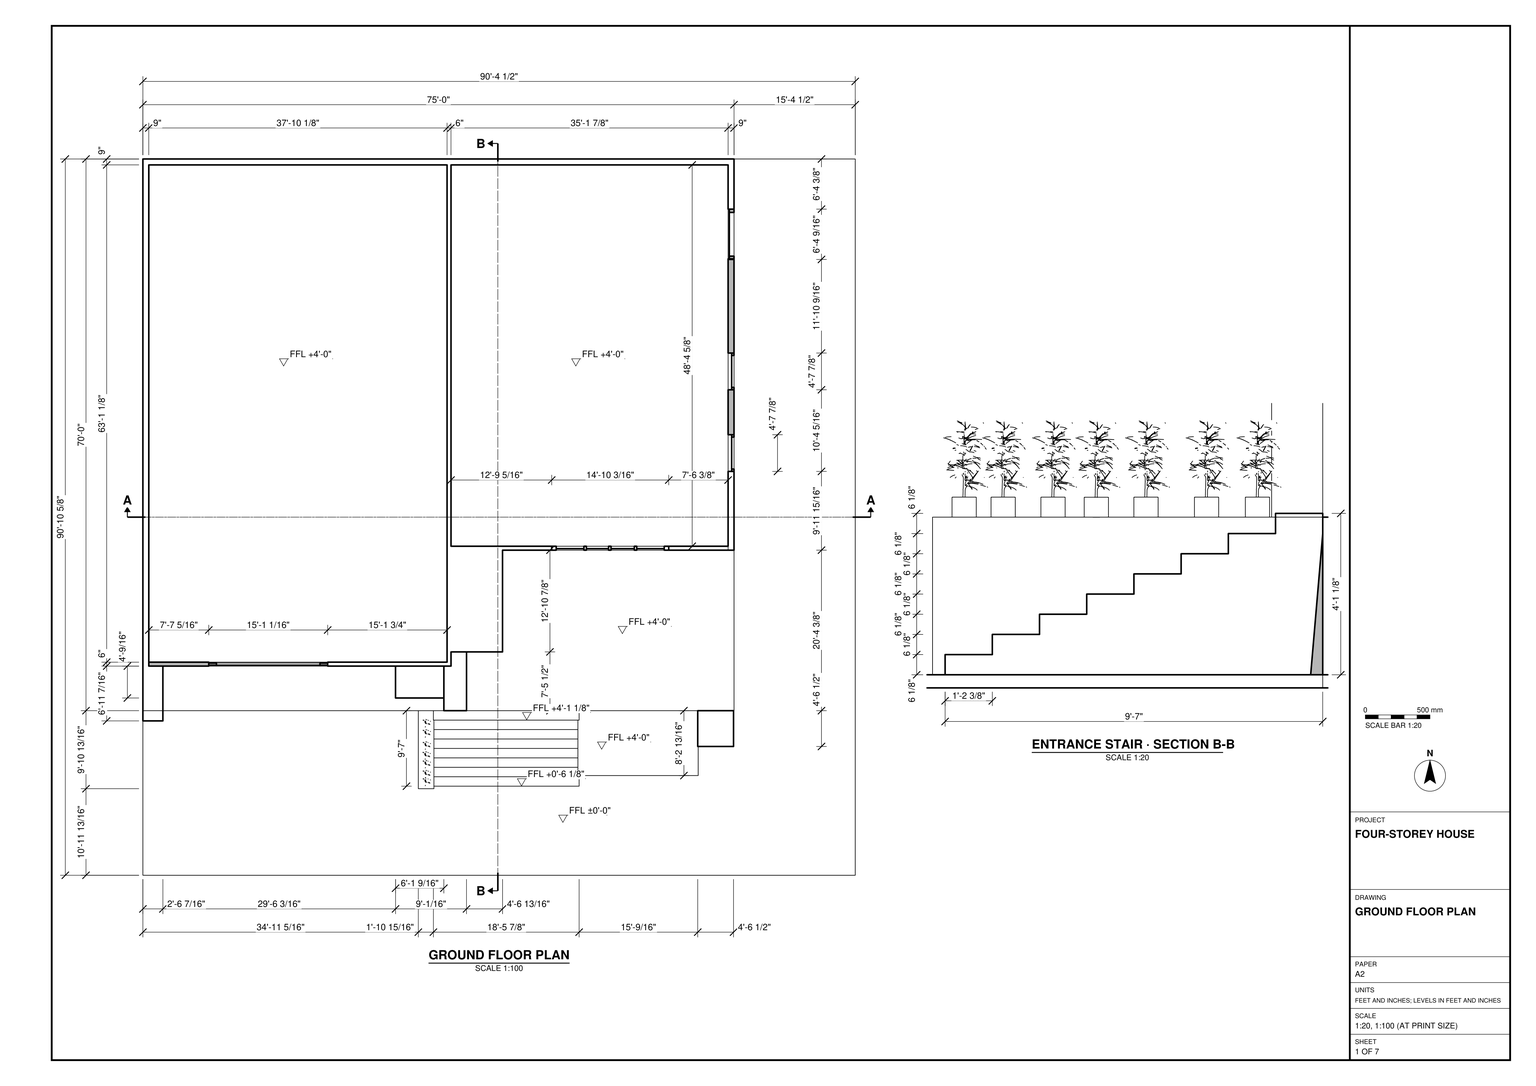
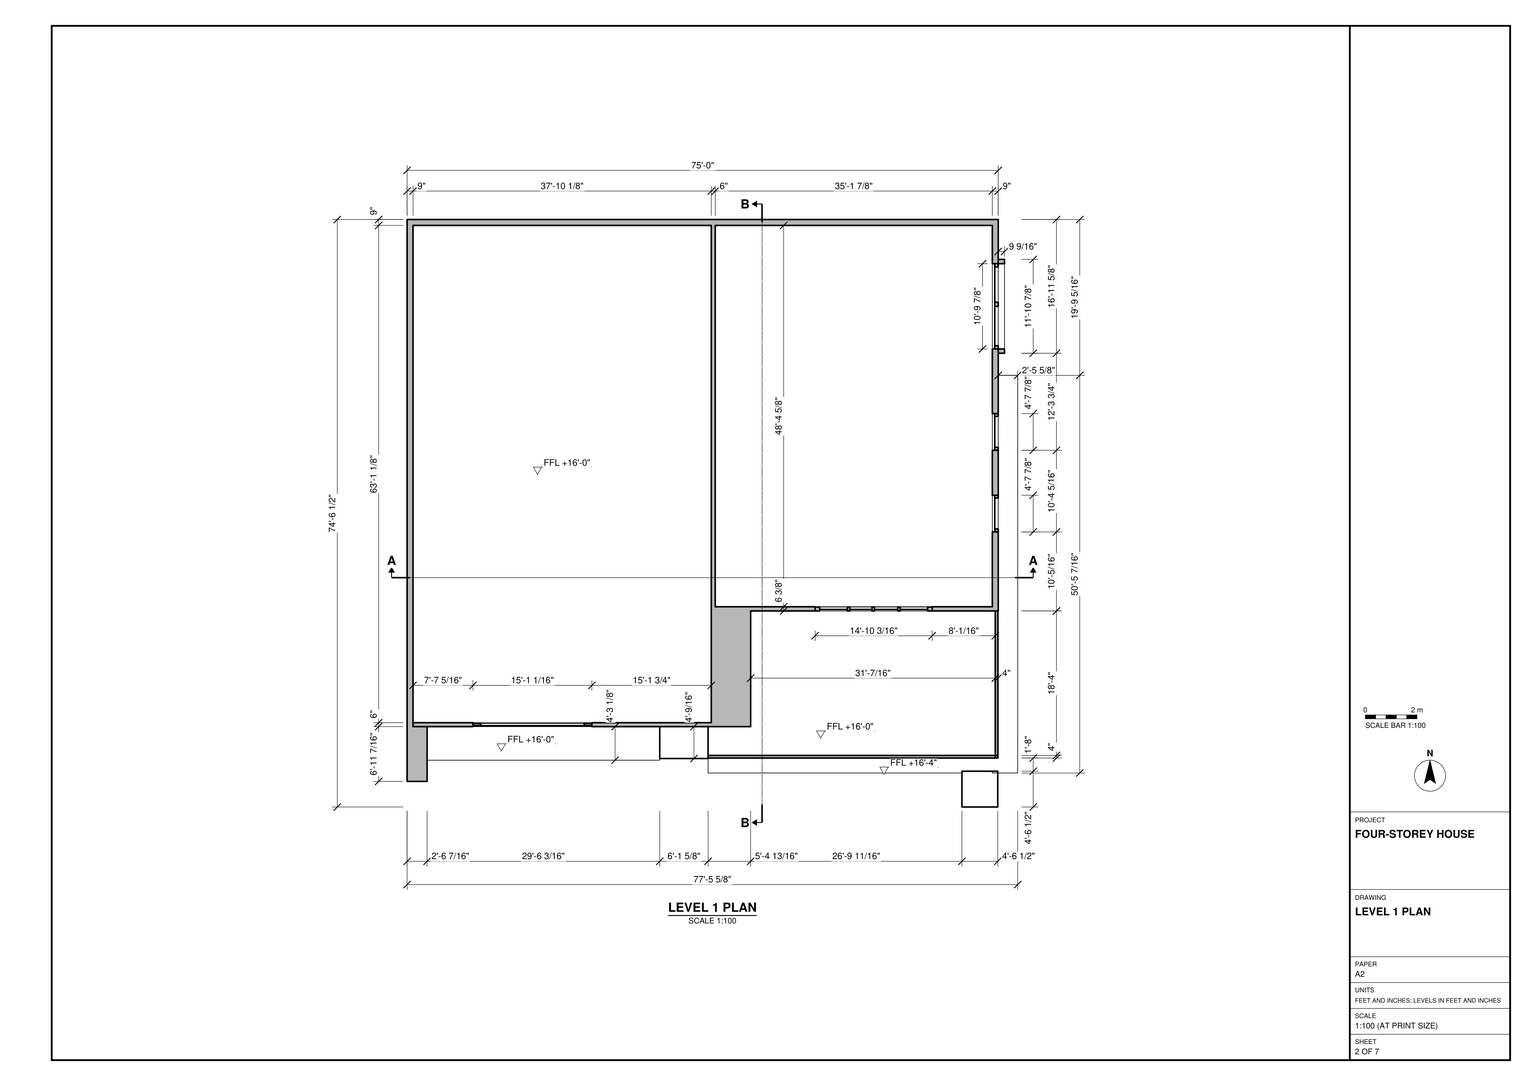
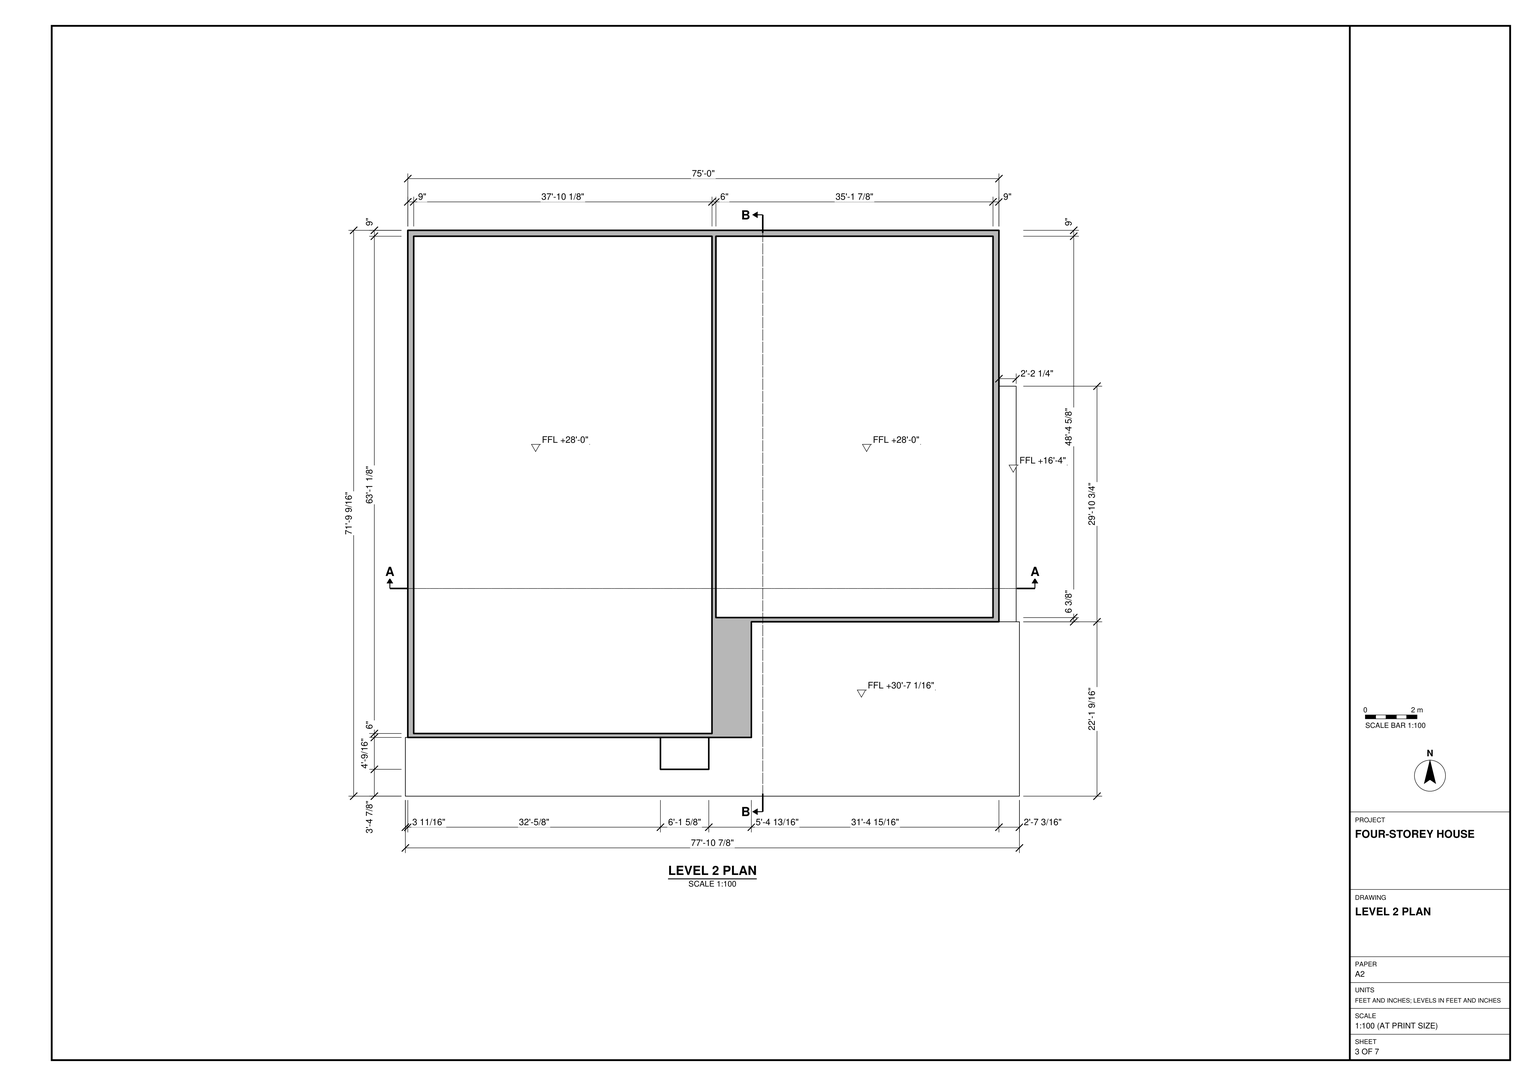
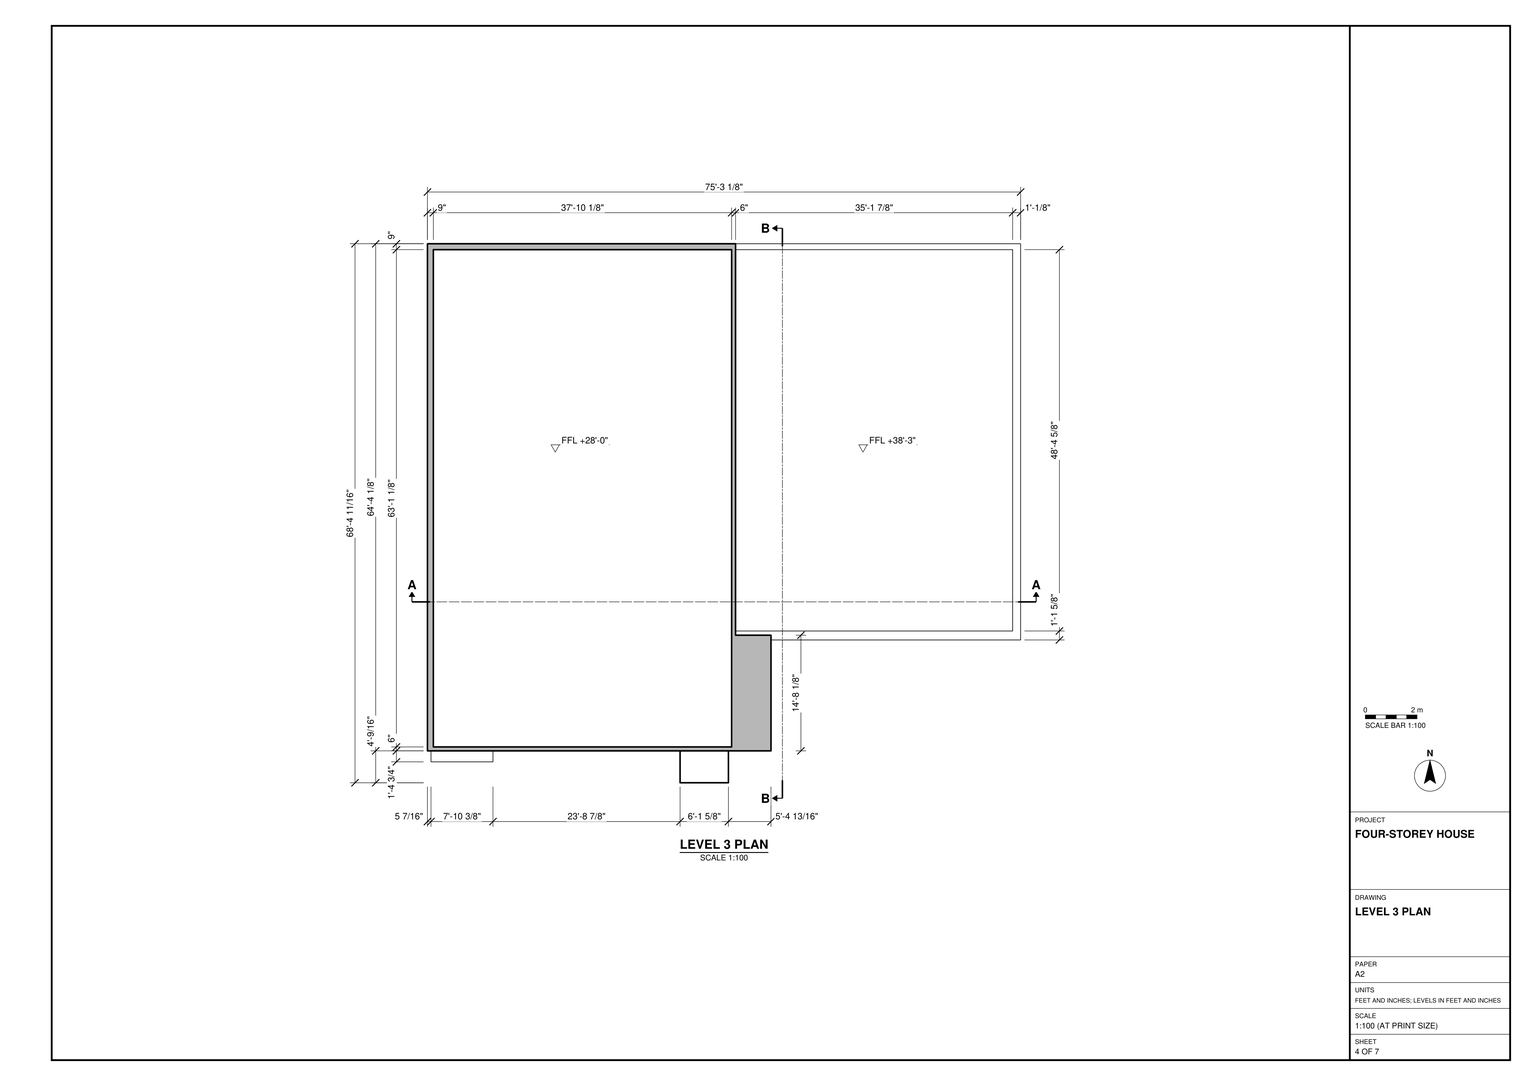
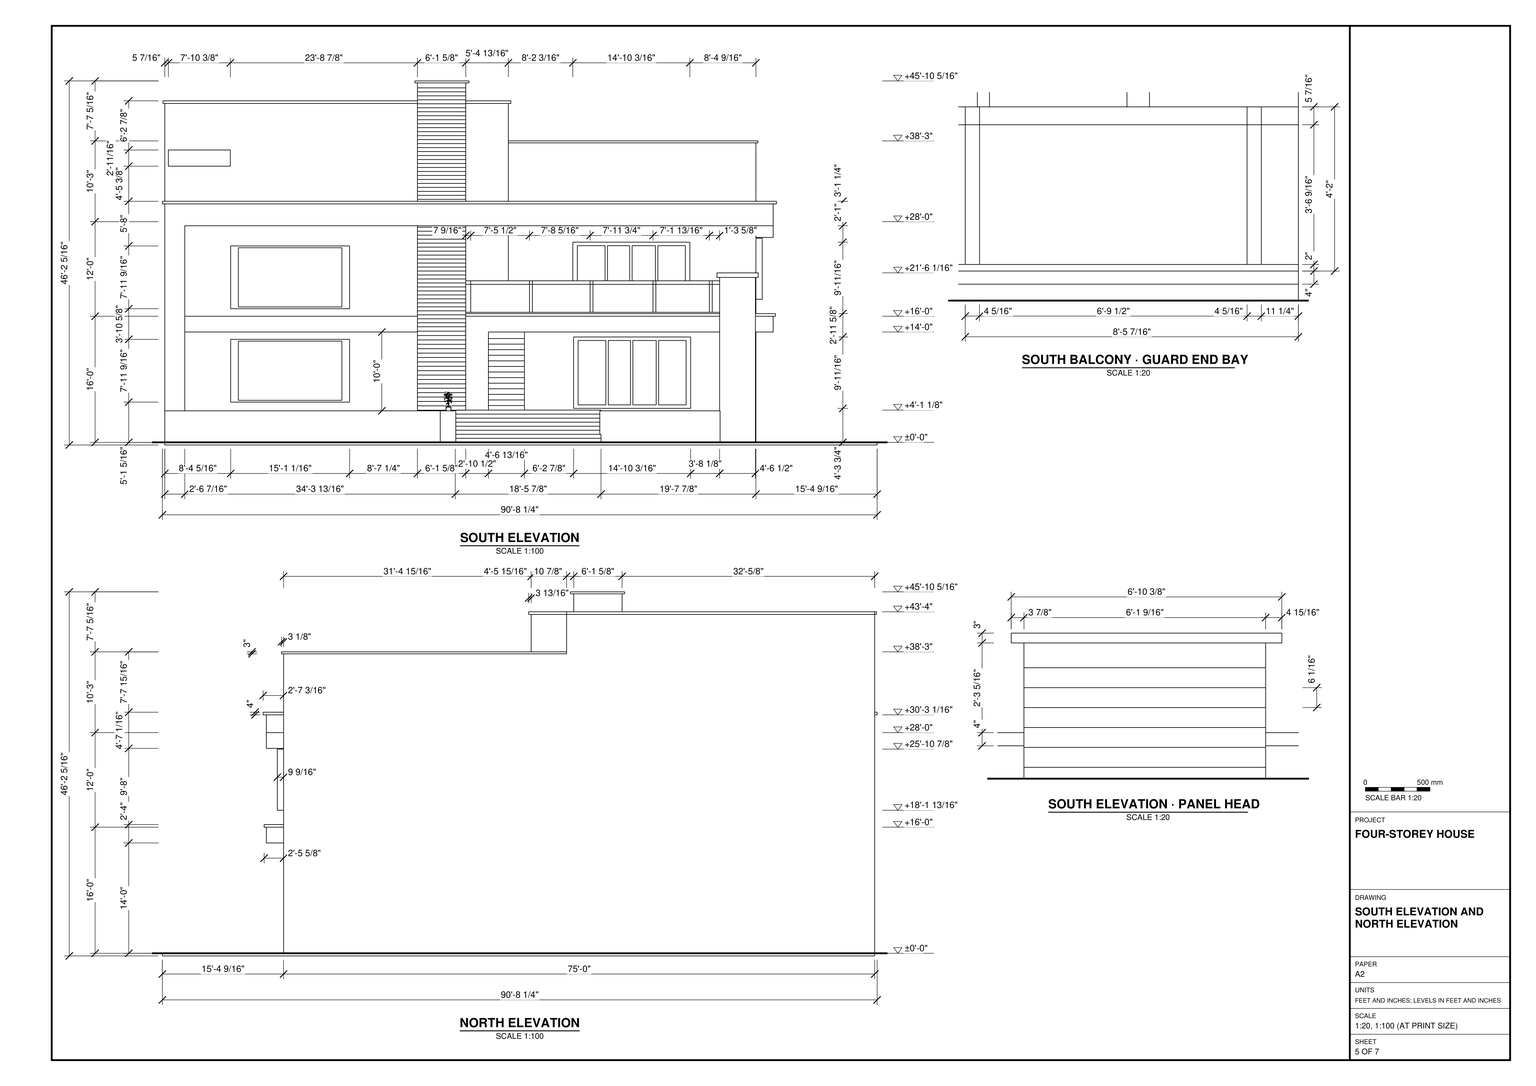
Build the four-storey house and its site in SketchUp from task_files/diagram_01.pdf. Work in feet and inches. Including the site, the model must measure 90'-8 1/4" along X, 90'-10 5/8" along Y and 46'-2 5/16" along Z. Use the level references ±0'-0", +16'-0", +28'-0" and +38'-3". Distinguish the ±0'-0" site datum from the raised ground-floor surface at +4'-0".

Align the two main bays along their rear wall, with the left bay extending farther toward the entrance than the right bay. Use the wall thicknesses shown, including the 9" rear wall and 6" dividing wall. Place the front and side openings in their dimensioned positions. Follow each floor plan for the slab edges, including the terrace in front of the recessed right bay at Level 1. Model the supports and roof to the profiles shown. Use section B-B to form the entrance stair and landing, and place the potted plants along the indicated edge of the stair.

Keep shell elements such as walls, slabs and roof, and each furniture or joinery piece shown, in separate groups or components. Use components for repeated parts. Decor and loose items, including the plants, may be any suitable library components. Save one SketchUp model as output_files/four_storey_house_with_a_raised_entrance.skp.

# SketchUp Ruby script. Lengths in inches.
U = 1.inch
M = Sketchup.active_model
def pt(a) = Geom::Point3d.new(a.map { |v| v * U })
def face(e, loops, mat)
  f = e.add_face(loops[0].map { |a| pt(a) })
  loops[1..].each { |l| e.add_face(l.map { |a| pt(a) }).erase! }
  f.material = f.back_material = mat if mat
  f
end
# faces: each face lists its corners as indices into pts; further lists are holes
def faces(e, pts, list, mat = nil) = list.each { |f| face(e, (f[0].is_a?(Array) ? f : [f]).map { |l| l.map { |i| pts[i] } }, mat) }
# xy, xz, yz: faces in a plane at the given z, y or x. An outline is a flat list of corners, or four numbers for a rectangle; further outlines are holes
def ring(l) = l.size == 4 ? [[l[0], l[1]], [l[2], l[1]], [l[2], l[3]], [l[0], l[3]]] : l.each_slice(2).to_a
def flat(e, list, mat, &to3) = list.each { |f| face(e, (f[0].is_a?(Array) ? f : [f]).map { |l| ring(l).map { |u, v| to3.(u, v) } }, mat) }
def xy(e, z, list, mat = nil) = flat(e, list, mat) { |x, y| [x, y, z] }
def xz(e, y, list, mat = nil) = flat(e, list, mat) { |x, z| [x, y, z] }
def yz(e, x, list, mat = nil) = flat(e, list, mat) { |y, z| [x, y, z] }
def lines(e, pts, list) = list.each { |a, b| e.add_line(pt(pts[a]), pt(pts[b])) }
# prism: a flat outline (further loops are holes) pulled along v
def prism(e, loops, v, mat = nil)
  f = face(e, loops, mat); d = Geom::Vector3d.new(v.map { |x| x * U })
  f.pushpull(f.normal.samedirection?(d) ? d.length : -d.length)
end
def box(e, o, s, mat = nil) = prism(e, [[o, [o[0] + s[0], o[1], o[2]], [o[0] + s[0], o[1] + s[1], o[2]], [o[0], o[1] + s[1], o[2]]]], [0, 0, s[2]], mat)
def at(x, y, z, deg = 0) = Geom::Transformation.translation(pt([x, y, z])) * Geom::Transformation.rotation(ORIGIN, Z_AXIS, deg.degrees)
def axes(o, x, y, z) = Geom::Transformation.new([*x, 0, *y, 0, *z, 0, *pt(o).to_a, 1])
def part(name) = M.definitions.add(name)
# library, detail: a bought-in or finely detailed component or shape, given as its bounding box
def library(name, o, s) = part(name).tap { |d| box(d.entities, o, s) }
def detail(e, o, s) = box(e.add_group.entities, o, s)
def put(e, d, t, mat = nil) = e.add_instance(d, t).tap { |i| i.material = mat if mat }
def group(e, t, mat = nil) = e.add_group.tap { |g| g.transformation = t; g.material = mat if mat }.entities
root = M.entities
M.materials.add("[Color B08]1").color = [50, 25, 0]
M.materials.add("[Color C08]").color = [60, 37, 47]
M.materials.add("[Color M04]").color = [142, 142, 142]
M.materials.add("[Color M05]").color = [114, 114, 114]
M.materials.add("[Color M06]").color = [86, 86, 86]
M.materials.add("[Color M07]").color = [58, 58, 58]
M.materials.add("[Concrete Block Retaining Gray]").color = [121, 121, 121]
M.materials.add("[Pavers with Grass Herringbone]").color = [197, 201, 190]
M.materials.add("[Translucent Glass Gray]").color = [128, 128, 128]
M.materials["[Translucent Glass Gray]"].alpha = 0.5
M.materials.add("[Wood Floor]").color = [155, 105, 61]
c1 = library("Potted plant",[-1.33,-1.39,0],[17.37,17.18,29.73])
c2 = part("Group\#1")
xy(c2.entities,0,[[0,0,156.875,9.8125]],"[Color B08]1")
xy(c2.entities,6.04,[[6.04,0,43.23,3.8125],[46.47,0,76.23,3.8125],[79.47,0,110.73,3.8125],[113.97,0,150.84,3.8125],[6.04,3.8125,43.23,9.8125],
  [46.47,3.8125,76.23,9.8125],[79.47,3.8125,110.73,9.8125],[113.97,3.8125,150.84,9.8125]],"[Color B08]1")
xy(c2.entities,116.59,[[6.04,0,43.23,3.8125],[46.47,0,76.23,3.8125],[79.47,0,110.73,3.8125],[113.97,0,150.84,3.8125],[6.04,3.8125,43.23,9.8125],
  [46.47,3.8125,76.23,9.8125],[79.47,3.8125,110.73,9.8125],[113.97,3.8125,150.84,9.8125]],"[Color B08]1")
xy(c2.entities,122.625,[[0,0,156.875,9.8125]],"[Color B08]1")
xz(c2.entities,0,[[[0,0,156.875,122.625],[6.04,6.04,43.23,116.59],[113.97,6.04,150.84,116.59],[79.47,6.04,110.73,116.59],[46.47,6.04,76.23,116.59]]],"[Color C08]")
xz(c2.entities,3.8125,[[6.04,6.04,43.23,116.59],[46.47,6.04,76.23,116.59],[79.47,6.04,110.73,116.59],[113.97,6.04,150.84,116.59]],"[Translucent Glass Gray]")
xz(c2.entities,9.8125,[[[0,0,156.875,122.625],[6.04,6.04,43.23,116.59],[113.97,6.04,150.84,116.59],[79.47,6.04,110.73,116.59],[46.47,6.04,76.23,116.59]]],"[Color B08]1")
yz(c2.entities,0,[[0,0,9.8125,122.625]],"[Color B08]1")
yz(c2.entities,6.04,[[0,6.04,3.8125,116.59],[3.8125,6.04,9.8125,116.59]],"[Color B08]1")
yz(c2.entities,43.23,[[0,6.04,3.8125,116.59]])
yz(c2.entities,43.23,[[3.8125,6.04,9.8125,116.59]],"[Color B08]1")
yz(c2.entities,46.47,[[0,6.04,3.8125,116.59],[3.8125,6.04,9.8125,116.59]],"[Color B08]1")
yz(c2.entities,76.23,[[0,6.04,3.8125,116.59]])
yz(c2.entities,76.23,[[3.8125,6.04,9.8125,116.59]],"[Color B08]1")
yz(c2.entities,79.47,[[0,6.04,3.8125,116.59],[3.8125,6.04,9.8125,116.59]],"[Color B08]1")
yz(c2.entities,110.73,[[0,6.04,3.8125,116.59]])
yz(c2.entities,110.73,[[3.8125,6.04,9.8125,116.59]],"[Color B08]1")
yz(c2.entities,113.97,[[0,6.04,3.8125,116.59],[3.8125,6.04,9.8125,116.59]],"[Color B08]1")
yz(c2.entities,150.84,[[0,6.04,3.8125,116.59]])
yz(c2.entities,150.84,[[3.8125,6.04,9.8125,116.59]],"[Color B08]1")
yz(c2.entities,156.875,[[0,0,9.8125,122.625]],"[Color B08]1")
c3 = part("Group\#2")
xy(c3.entities,0,[[0,0,57.0625,5.875]],"[Color B08]1")
xy(c3.entities,3.7,[[3.7,0,53.36,5.875]],"[Color B08]1")
xy(c3.entities,127.24,[[3.7,0,53.36,5.875]],"[Color B08]1")
xy(c3.entities,130.9375,[[0,0,57.0625,5.875]],"[Color B08]1")
xz(c3.entities,0,[[[0,0,57.0625,130.9375],[3.7,3.7,53.36,127.24]]],"[Color B08]1")
xz(c3.entities,5.875,[[[0,0,57.0625,130.9375],[3.7,3.7,53.36,127.24]]],"[Color B08]1")
xz(c3.entities,5.875,[[3.7,3.7,53.36,127.24]],"[Translucent Glass Gray]")
yz(c3.entities,0,[[0,0,5.875,130.9375]],"[Color B08]1")
yz(c3.entities,3.7,[[0,3.7,5.875,127.24]],"[Color B08]1")
yz(c3.entities,53.36,[[0,3.7,5.875,127.24]],"[Color B08]1")
yz(c3.entities,57.0625,[[0,0,5.875,130.9375]],"[Color B08]1")
c4 = part("Group\#3")
xy(c4.entities,0,[[0,0,69.8125,7.4375]],"[Color B08]1")
xy(c4.entities,5.34,[[5.34,0,64.47,7.4375]],"[Color B08]1")
xy(c4.entities,71.03,[[5.34,0,64.47,7.4375]],"[Color B08]1")
xy(c4.entities,77.875,[[5.34,0,64.47,7.4375]],"[Color B08]1")
xy(c4.entities,136.79,[[5.34,0,64.47,7.4375]],"[Color B08]1")
xy(c4.entities,142.125,[[0,0,69.8125,7.4375]],"[Color B08]1")
xz(c4.entities,0,[[[0,0,69.8125,142.125],[5.34,5.34,64.47,71.03],[5.34,77.875,64.47,136.79]]],"[Color B08]1")
xz(c4.entities,7.4375,[[[0,0,69.8125,142.125],[5.34,5.34,64.47,71.03],[5.34,77.875,64.47,136.79]]],"[Color B08]1")
xz(c4.entities,7.4375,[[5.34,5.34,64.47,71.03],[5.34,77.875,64.47,136.79]],"[Translucent Glass Gray]")
yz(c4.entities,0,[[0,0,7.4375,142.125]],"[Color B08]1")
yz(c4.entities,5.34,[[0,5.34,7.4375,71.03],[0,77.875,7.4375,136.79]],"[Color B08]1")
yz(c4.entities,64.47,[[0,5.34,7.4375,71.03],[0,77.875,7.4375,136.79]],"[Color B08]1")
yz(c4.entities,69.8125,[[0,0,7.4375,142.125]],"[Color B08]1")
xy(root,-4,[[3.6875,0,1088.25,250.625],[3.6875,250.625,1088.25,1090.625]])
xy(root,0,[[848.44,196.125,849.14,250.625],[849.14,196.125,902.94,250.625],[3.6875,250.625,903.6875,1090.625]])
xy(root,0,[[423.05,131.8125,446.8,250.625],[666.02,151.8125,666.02,250.625,848.44,250.625,848.44,196.125,849.14,196.125,849.14,151.8125]],"[Concrete Block Retaining Gray]")
xy(root,0,[[3.6875,0,1088.25,0,1088.25,1090.625,903.6875,1090.625,903.6875,250.625,902.94,250.625,902.94,196.125,849.14,196.125,849.14,151.8125,666.02,151.8125,666.02,250.625,446.8,250.625,446.8,131.8125,423.05,131.8125,423.05,250.625,3.6875,250.625]],"[Pavers with Grass Herringbone]")
xy(root,48,[[3.6875,235.0625,34.125,250.625],[34.125,250.625,461.9375,250.625,461.9375,269.9375,388.33,269.9375,388.33,318.5,34.125,318.5],[461.9375,250.625,461.9375,318.5,472.8125,318.5,472.8125,340.125,496.4375,340.125,496.4375,250.625],[496.4375,250.625,903.6875,250.625,903.6875,495,551.25,495,551.25,340.125,496.4375,340.125],[12.6875,324.5,466.8125,1081.625],
  [894.6875,495,903.6875,690.86],[472.8125,501,894.6875,1081.625],[894.6875,690.86,903.6875,733.96]])
xy(root,48,[[423.05,131.8125,446.8,250.625],[666.02,151.8125,849.14,151.8125,849.14,196.125,848.44,196.125,848.44,250.625,666.02,250.625]],"[Concrete Block Retaining Gray]")
xy(root,51.76,[[626.11,495,804.29,501]])
xy(root,54.02,[[894.6875,614.93,903.6875,670.8],[894.6875,739.24,903.6875,795.12]])
xy(root,54.63,[[894.6875,938.625,903.6875,1014.25]])
xy(root,61.29,[[104,318.5,285.0625,324.5]])
xy(root,156.86,[[104,318.5,285.0625,324.5]])
xy(root,159.21,[[894.6875,614.93,903.6875,670.8],[894.6875,670.8,903.6875,739.24],[894.6875,739.24,903.6875,795.12]])
xy(root,160.45,[[626.11,495,804.29,501]])
xy(root,161.63,[[894.6875,938.625,903.6875,1014.25]])
xy(root,168,[[894.6875,250.0625,894.6875,250.625,496.4375,250.625,496.4375,340.125,551.25,340.125,551.25,495,903.6875,495,903.6875,853.33,929.9375,853.33,929.9375,250.0625]])
xy(root,168,[[34.125,267.375,388.33,318.5]],"[Color M07]")
xy(root,192,[[894.6875,250.0625,894.6875,250.625,461.9375,250.625,461.9375,270.625,903.1875,270.625,903.1875,494.61,903.6875,494.61,903.6875,853.33,929.9375,853.33,929.9375,250.0625],[461.9375,270.625,899.1875,274.625],[461.9375,274.625,899.1875,274.625,899.1875,494.61,526.75,494.61,526.75,318.5,461.9375,318.5],[12.6875,324.5,466.8125,1081.625],[472.8125,501,894.6875,1081.625]])
xy(root,192,[[929.9375,247.875,933.3125,853.33]],"[Color M06]")
xy(root,192,[[461.9375,247.875,848.44,250.625],[894.6875,247.875,929.9375,250.0625],[34.125,267.375,388.33,318.5]],"[Color M07]")
xy(root,196,[[461.9375,247.875,848.44,247.875,848.44,250.625,894.6875,250.625,894.6875,247.875,933.3125,247.875,933.3125,853.33,903.6875,853.33,903.6875,494.61,903.1875,494.61,903.1875,270.625,461.9375,270.625]],"[Color M07]")
xy(root,196.1,[[624.92,494.61,803.11,501]])
xy(root,197.875,[[899.1875,270.625,903.1875,274.625],[899.1875,274.625,903.1875,494.61]])
xy(root,198,[[461.9375,270.625,899.1875,274.625]])
xy(root,200.96,[[894.6875,614.93,903.6875,670.8],[894.6875,739.24,903.6875,795.12]])
xy(root,203.48,[[104,318.5,285.0625,324.5]])
xy(root,217.8,[[903.6875,887,913.25,1029.9]],"[Color M06]")
xy(root,227.69,[[894.6875,893.51,903.6875,1023.38]])
xy(root,227.69,[[903.6875,893.51,913.25,1023.38]],"[Color M06]")
xy(root,246,[[461.9375,270.625,469.47,274.625]])
xy(root,246,[[469.47,270.625,558.95,274.625],[558.95,270.625,563.3,274.625],[563.3,270.625,651.26,274.625],[651.26,270.625,655.61,274.625],[655.61,270.625,747.01,274.625],
  [747.01,270.625,751.36,274.625],[751.36,270.625,832.82,274.625],[832.82,270.625,837.17,274.625],[837.17,270.625,899.1875,274.625],[899.1875,270.625,903.1875,274.625],
  [899.1875,274.625,903.1875,321.65],[899.1875,321.65,903.1875,325.66],[899.1875,325.66,903.1875,383.96],[899.1875,383.96,903.1875,387.97],[899.1875,387.97,903.1875,439.9],
  [899.1875,439.9,903.1875,443.91],[899.1875,443.91,903.1875,494.61]],"[Color B08]1")
xy(root,251.125,[[848.44,196.125,902.94,250.625]])
xy(root,251.125,[[844.38,192.5625,844.38,250.625,848.44,250.625,848.44,196.125,902.94,196.125,902.94,250.625,907.19,250.625,907.19,192.5625]],"[Color M07]")
xy(root,258.0625,[[844.38,192.5625,907.19,250.625]],"[Color M07]")
xy(root,299,[[894.6875,893.51,903.6875,1023.38]])
xy(root,299,[[903.6875,893.51,913.25,1023.38]],"[Color M06]")
xy(root,299.04,[[104,318.5,285.0625,324.5]])
xy(root,303.89,[[894.6875,614.93,903.6875,670.8],[894.6875,739.24,903.6875,795.12]])
xy(root,304.79,[[624.92,494.61,803.11,501]])
xy(root,310.88,[[903.6875,887,913.25,1029.9]],"[Color M06]")
xy(root,312,[[903.6875,494.61,929.9375,853.33]])
xy(root,329.8125,[[34.125,235.0625,34.125,318.5,388.33,318.5,388.33,269.9375,461.9375,269.9375,461.9375,318.5,526.75,318.5,526.75,494.61,929.9375,494.61,929.9375,235.0625]])
xy(root,336,[[12.6875,324.5,466.8125,1081.625],[472.8125,501,894.6875,1081.625]])
xy(root,336,[[903.6875,494.61,929.9375,853.33]],"[Color M06]")
xy(root,363.0625,[[3.6875,235.0625,3.6875,318.5,388.33,318.5,388.33,269.9375,461.9375,269.9375,461.9375,318.5,526.75,318.5,526.75,494.61,929.9375,494.61,929.9375,235.0625]])
xy(root,363.0625,[[0,229.0625,0,318.5,3.6875,318.5,3.6875,235.0625,929.9375,235.0625,929.9375,494.61,934.875,494.61,934.875,229.0625]],"[Color M07]")
xy(root,367.0625,[[472.8125,318.5,526.75,494.61]])
xy(root,367.0625,[[0,229.0625,934.875,229.0625,934.875,494.61,526.75,494.61,526.75,318.5,461.9375,318.5,461.9375,269.9375,388.33,269.9375,388.33,318.5,0,318.5]],"[Color M05]")
xy(root,420.47,[[9.11,301.75,103.48,318.5]],"[Color M07]")
xy(root,445.16,[[9.11,301.75,103.48,318.5]],"[Color M07]")
xy(root,456,[[472.8125,494.61,472.8125,501,894.6875,501,894.6875,1081.625,472.8125,1081.625,472.8125,1090.625,903.6875,1090.625,903.6875,494.61],[903.6875,494.61,906.8125,1090.625]])
xy(root,456,[[526.75,487.36,906.8125,494.61]],"[Color M07]")
xy(root,459,[[526.75,487.36,906.8125,487.36,906.8125,1090.625,472.8125,1090.625,472.8125,1081.625,894.6875,1081.625,894.6875,501,472.8125,501,472.8125,494.61,526.75,494.61],[472.8125,501,894.6875,1081.625]],"[Color M07]")
xy(root,516,[[0.9375,314.875,3.6875,1090.625],[3.6875,314.875,388.33,318.5],[[3.6875,318.5,3.6875,1090.625,472.8125,1090.625,472.8125,494.61,526.75,494.61,526.75,318.5],[12.6875,324.5,466.8125,1081.625]]])
xy(root,516,[[461.9375,314.875,461.9375,318.5,526.75,318.5,526.75,494.61,530.5625,494.61,530.5625,314.875]],"[Color M07]")
xy(root,520,[[0.9375,314.875,388.33,314.875,388.33,318.5,461.9375,318.5,461.9375,314.875,530.5625,314.875,530.5625,494.61,472.8125,494.61,472.8125,1090.625,0.9375,1090.625]],"[Color M07]")
xy(root,547.3125,[[388.33,269.9375,461.9375,318.5]])
xy(root,547.3125,[[384.45,266.125,466.875,269.9375],[384.45,269.9375,388.33,318.5],[461.9375,269.9375,466.875,318.5]],"[Color M05]")
xy(root,550.3125,[[384.45,266.125,466.875,318.5]],"[Color M05]")
xz(root,0,[[3.6875,-4,1088.25,0]])
xz(root,131.8125,[[423.05,0,446.8,48]],"[Concrete Block Retaining Gray]")
xz(root,151.8125,[[666.02,0,849.14,48]],"[Concrete Block Retaining Gray]")
xz(root,192.5625,[[844.38,251.125,907.19,258.0625]],"[Color M07]")
xz(root,196.125,[[849.14,0,902.94,0,902.94,251.125,848.44,251.125,848.44,48,849.14,48]],"[Color M06]")
xz(root,196.125,[[848.44,0,849.14,48]],"[Concrete Block Retaining Gray]")
xz(root,229.0625,[[0,363.0625,934.875,367.0625]],"[Color M07]")
xz(root,235.0625,[[3.6875,48,34.125,48,34.125,329.8125,929.9375,329.8125,929.9375,363.0625,3.6875,363.0625]],"[Color M06]")
xz(root,247.875,[[461.9375,192,848.44,196],[894.6875,192,933.3125,196]],"[Color M07]")
xz(root,250.0625,[[894.6875,168,929.9375,192]],"[Color M06]")
xz(root,250.625,[[848.44,0,902.94,48],[902.94,0,903.6875,48],[848.44,168,894.6875,192],[848.44,192,894.6875,196],[844.38,251.125,907.19,258.0625]])
xz(root,250.625,[[461.9375,48,496.4375,48,496.4375,168,848.44,168,848.44,192,461.9375,192],[848.44,48,848.44,168,894.6875,168,894.6875,196,848.44,196,848.44,251.125,902.94,251.125,902.94,48]],"[Color M06]")
xz(root,250.625,[[3.6875,0,423.05,48],[446.8,0,666.02,48]],"[Color M07]")
xz(root,250.625,[[423.05,0,446.8,48],[666.02,0,848.44,48]],"[Concrete Block Retaining Gray]")
xz(root,266.125,[[384.45,547.3125,466.875,550.3125]],"[Color M05]")
xz(root,267.375,[[34.125,168,388.33,192]],"[Color M07]")
xz(root,269.9375,[[388.33,329.8125,461.9375,333.63],[388.33,333.63,461.9375,339.69],[388.33,339.69,461.9375,345.76],[388.33,345.76,461.9375,351.82],[388.33,351.82,461.9375,357.88],
  [388.33,357.88,461.9375,363.0625],[388.33,363.0625,461.9375,363.94],[388.33,363.94,461.9375,367.0625]])
xz(root,269.9375,[[388.33,48,461.9375,48.94],[388.33,48.94,461.9375,55.63],[388.33,55.63,461.9375,62.32],[388.33,62.32,461.9375,69.01],[388.33,69.01,461.9375,75.69],
  [388.33,75.69,461.9375,82.38],[388.33,82.38,461.9375,89.07],[388.33,89.07,461.9375,95.76],[388.33,95.76,461.9375,102.44],[388.33,102.44,461.9375,109.13],
  [388.33,109.13,461.9375,115.82],[388.33,115.82,461.9375,122.51],[388.33,122.51,461.9375,129.19],[388.33,129.19,461.9375,135.88],[388.33,135.88,461.9375,142.57],
  [388.33,142.57,461.9375,149.26],[388.33,149.26,461.9375,155.94],[388.33,155.94,461.9375,162.63],[388.33,162.63,461.9375,169.32],[388.33,169.32,461.9375,176.01],
  [388.33,176.01,461.9375,182.07],[388.33,182.07,461.9375,188.13],[388.33,188.13,461.9375,194.19],[388.33,194.19,461.9375,200.26],[388.33,200.26,461.9375,206.32],
  [388.33,206.32,461.9375,212.38],[388.33,212.38,461.9375,218.44],[388.33,218.44,461.9375,224.51],[388.33,224.51,461.9375,230.57],[388.33,230.57,461.9375,236.63],
  [388.33,236.63,461.9375,242.69],[388.33,242.69,461.9375,248.76],[388.33,248.76,461.9375,254.82],[388.33,254.82,461.9375,260.88],[388.33,260.88,461.9375,266.94],
  [388.33,266.94,461.9375,273.01],[388.33,273.01,461.9375,279.07],[388.33,279.07,461.9375,285.13],[388.33,285.13,461.9375,291.19],[388.33,291.19,461.9375,297.26],
  [388.33,297.26,461.9375,303.32],[388.33,303.32,461.9375,309.38],[388.33,309.38,461.9375,315.44],[388.33,315.44,461.9375,321.51],[388.33,321.51,461.9375,327.57],
  [388.33,327.57,461.9375,329.8125],[388.33,367.0625,461.9375,370.01],[388.33,370.01,461.9375,376.07],[388.33,376.07,461.9375,382.13],[388.33,382.13,461.9375,388.19],
  [388.33,388.19,461.9375,394.26],[388.33,394.26,461.9375,400.32],[388.33,400.32,461.9375,406.38],[388.33,406.38,461.9375,412.44],[388.33,412.44,461.9375,418.51],
  [388.33,418.51,461.9375,424.57],[388.33,424.57,461.9375,430.63],[388.33,430.63,461.9375,436.69],[388.33,436.69,461.9375,442.76],[388.33,442.76,461.9375,448.82],
  [388.33,448.82,461.9375,454.88],[388.33,454.88,461.9375,460.94],[388.33,460.94,461.9375,467.01],[388.33,467.01,461.9375,473.07],[388.33,473.07,461.9375,479.13],
  [388.33,479.13,461.9375,485.19],[388.33,485.19,461.9375,491.26],[388.33,491.26,461.9375,497.32],[388.33,497.32,461.9375,503.38],[388.33,503.38,461.9375,509.44],
  [388.33,509.44,461.9375,515.51],[388.33,515.51,461.9375,521.57],[388.33,521.57,461.9375,527.63],[388.33,527.63,461.9375,533.69],[388.33,533.69,461.9375,539.76],
  [388.33,539.76,461.9375,547.3125]],"[Wood Floor]")
xz(root,270.625,[[461.9375,192,899.1875,196],[899.1875,192,903.1875,196]])
xz(root,270.625,[[461.9375,196,899.1875,198],[899.1875,196,903.1875,197.875],[899.1875,197.875,903.1875,240.56],[461.9375,198,469.47,240.56],[558.95,198,563.3,240.56],
  [651.26,198,655.61,240.56],[747.01,198,751.36,240.56],[832.82,198,837.17,240.56],[461.9375,240.56,469.47,246],[469.47,240.56,558.95,246],
  [558.95,240.56,563.3,246],[563.3,240.56,651.26,246],[651.26,240.56,655.61,246],[655.61,240.56,747.01,246],[747.01,240.56,751.36,246],
  [751.36,240.56,832.82,246],[832.82,240.56,837.17,246],[837.17,240.56,899.1875,246],[899.1875,240.56,903.1875,246]],"[Color B08]1")
xz(root,270.625,[[469.47,198,558.95,240.56],[563.3,198,651.26,240.56],[655.61,198,747.01,240.56],[751.36,198,832.82,240.56],[837.17,198,899.1875,240.56]],"[Translucent Glass Gray]")
xz(root,274.625,[[899.1875,197.875,903.1875,246]])
xz(root,274.625,[[461.9375,192,899.1875,198],[461.9375,198,469.47,241.64],[558.95,198,563.3,241.64],[651.26,198,655.61,241.64],[747.01,198,751.36,241.64],
  [832.82,198,837.17,241.64],[893.13,198,899.1875,241.64],[461.9375,241.64,469.47,246],[469.47,241.64,558.95,246],[558.95,241.64,563.3,246],
  [563.3,241.64,651.26,246],[651.26,241.64,655.61,246],[655.61,241.64,747.01,246],[747.01,241.64,751.36,246],[751.36,241.64,832.82,246],
  [832.82,241.64,837.17,246],[837.17,241.64,899.1875,246]],"[Color B08]1")
xz(root,274.625,[[469.47,198,558.95,241.64],[563.3,198,651.26,241.64],[655.61,198,747.01,241.64],[751.36,198,832.82,241.64],[837.17,198,893.13,241.64]],"[Translucent Glass Gray]")
xz(root,301.75,[[9.11,420.47,103.48,445.16]],"[Color M07]")
xz(root,314.875,[[0.9375,516,388.33,520],[461.9375,516,530.5625,520]],"[Color M07]")
xz(root,318.5,[[12.6875,48,34.125,168],[388.33,48,461.9375,168],[461.9375,48,472.8125,168],[12.6875,168,34.125,192],[388.33,168,461.9375,192],
  [12.6875,192,34.125,312],[388.33,192,461.9375,312],[12.6875,312,34.125,329.8125],[388.33,312,461.9375,336],[388.33,336,461.9375,456],
  [0,363.0625,3.6875,367.0625],[3.6875,363.0625,388.33,367.0625],[461.9375,363.0625,472.8125,367.0625],[472.8125,363.0625,526.75,367.0625],[388.33,456,461.9375,516],
  [388.33,516,461.9375,520],[388.33,520,461.9375,547.3125]])
xz(root,318.5,[[384.45,547.3125,466.875,550.3125]],"[Color M05]")
xz(root,318.5,[[[34.125,48,388.33,168],[104,61.29,285.0625,156.86]],[[34.125,192,388.33,329.8125],[104,203.48,285.0625,299.04]],[461.9375,192,526.75,329.8125],[[3.6875,367.0625,388.33,516],[9.11,420.47,103.48,445.16]],[461.9375,367.0625,526.75,516]],"[Color M07]")
xz(root,324.5,[[[12.6875,48,466.8125,168],[104,61.29,285.0625,156.86]],[12.6875,168,466.8125,192],[[12.6875,192,466.8125,312],[104,203.48,285.0625,299.04]],[12.6875,312,466.8125,336],[12.6875,336,466.8125,456],
  [12.6875,456,466.8125,516]])
xz(root,340.125,[[472.8125,48,496.4375,168]])
xz(root,340.125,[[496.4375,48,551.25,56.08],[496.4375,56.08,551.25,64.58],[496.4375,64.58,551.25,73.08],[496.4375,73.08,551.25,81.58],[496.4375,81.58,551.25,90.08],
  [496.4375,90.08,551.25,98.58],[496.4375,98.58,551.25,107.08],[496.4375,107.08,551.25,115.58],[496.4375,115.58,551.25,124.08],[496.4375,124.08,551.25,132.58],
  [496.4375,132.58,551.25,141.08],[496.4375,141.08,551.25,149.58],[496.4375,149.58,551.25,158.08],[496.4375,158.08,551.25,168]],"[Wood Floor]")
xz(root,487.36,[[526.75,456,906.8125,459]],"[Color M07]")
xz(root,494.61,[[899.1875,192,903.1875,197.875],[903.1875,192,903.6875,196],[899.1875,197.875,903.1875,246],[472.8125,312,472.8125,367.0625,526.75,367.0625,526.75,363.0625,903.6875,363.0625,903.6875,336,929.9375,336,929.9375,329.8125,526.75,329.8125,526.75,312],[526.75,363.0625,894.6875,367.0625],
  [894.6875,363.0625,903.6875,367.0625],[472.8125,456,526.75,459]])
xz(root,494.61,[[[526.75,192,899.1875,192,899.1875,246,903.1875,246,903.1875,196,903.6875,196,903.6875,329.8125,526.75,329.8125],[624.92,196.1,803.11,304.79]],[903.6875,336,929.9375,363.0625],[526.75,367.0625,903.6875,456]],"[Color M06]")
xz(root,494.61,[[903.6875,312,929.9375,329.8125],[903.6875,363.0625,934.875,367.0625],[472.8125,459,526.75,516],[472.8125,516,530.5625,520]],"[Color M07]")
xz(root,495,[[[551.25,48,903.6875,168],[626.11,51.76,804.29,160.45]]],"[Color M06]")
xz(root,501,[[[472.8125,48,894.6875,168],[626.11,51.76,804.29,160.45]],[472.8125,168,894.6875,192],[[472.8125,192,894.6875,312],[624.92,196.1,803.11,304.79]],[472.8125,312,894.6875,336],[472.8125,336,894.6875,456],
  [472.8125,456,894.6875,459]])
xz(root,614.93,[[894.6875,54.02,903.6875,159.21],[894.6875,200.96,903.6875,303.89]])
xz(root,670.8,[[894.6875,54.02,903.6875,159.21],[894.6875,200.96,903.6875,303.89]])
xz(root,739.24,[[894.6875,54.02,903.6875,159.21],[894.6875,200.96,903.6875,303.89]])
xz(root,795.12,[[894.6875,54.02,903.6875,159.21],[894.6875,200.96,903.6875,303.89]])
xz(root,853.33,[[903.6875,168,929.9375,192],[903.6875,312,929.9375,336]],"[Color M06]")
xz(root,853.33,[[903.6875,192,933.3125,196]],"[Color M07]")
xz(root,887,[[903.6875,217.8,913.25,310.88]],"[Color M06]")
xz(root,893.51,[[894.6875,227.69,903.6875,299]])
xz(root,893.51,[[903.6875,227.69,913.25,299]],"[Color M06]")
xz(root,938.625,[[894.6875,54.63,903.6875,161.63]])
xz(root,1014.25,[[894.6875,54.63,903.6875,161.63]])
xz(root,1023.38,[[894.6875,227.69,903.6875,299]])
xz(root,1023.38,[[903.6875,227.69,913.25,299]],"[Color M06]")
xz(root,1029.9,[[903.6875,217.8,913.25,310.88]],"[Color M06]")
xz(root,1081.625,[[12.6875,48,466.8125,168],[472.8125,48,894.6875,168],[12.6875,168,466.8125,192],[472.8125,168,894.6875,192],[12.6875,192,27.5625,312],
  [27.5625,192,466.8125,312],[472.8125,192,493.125,312],[493.125,192,894.6875,312],[12.6875,312,27.5625,336],[27.5625,312,466.8125,336],
  [472.8125,312,493.125,336],[493.125,312,894.6875,336],[12.6875,336,27.5625,456],[27.5625,336,466.8125,456],[472.8125,336,493.125,456],
  [493.125,336,894.6875,456],[12.6875,456,27.5625,516],[27.5625,456,466.8125,516],[472.8125,456,493.125,459],[493.125,456,894.6875,459]])
xz(root,1090.625,[[3.6875,-4,1088.25,0],[0.9375,516,3.6875,520]])
xz(root,1090.625,[[3.6875,0,3.6875,516,472.8125,516,472.8125,456,903.6875,456,903.6875,0],[472.8125,456,906.8125,459],[3.6875,516,472.8125,520]],"[Color M07]")
yz(root,0,[[229.0625,363.0625,318.5,367.0625]],"[Color M07]")
yz(root,0.9375,[[314.875,516,1090.625,520]],"[Color M07]")
yz(root,3.6875,[[0,-4,250.625,0],[250.625,-4,1090.625,0]])
yz(root,3.6875,[[250.625,0,1090.625,48],[235.0625,48,235.0625,363.0625,318.5,363.0625,318.5,516,1090.625,516,1090.625,48]],"[Color M07]")
yz(root,9.11,[[301.75,420.47,318.5,445.16]],"[Color M07]")
yz(root,12.6875,[[318.5,48,324.5,168],[324.5,48,1081.625,168],[318.5,168,324.5,192],[324.5,168,1081.625,192],[318.5,192,324.5,312],
  [324.5,192,1081.625,312],[318.5,312,318.5,329.8125,259.625,329.8125,259.625,336,324.5,336,324.5,312],[324.5,312,1081.625,336],[324.5,336,1081.625,456],[324.5,456,1081.625,516]])
yz(root,34.125,[[235.0625,48,318.5,48,318.5,168,267.375,168,267.375,192,318.5,192,318.5,329.8125,235.0625,329.8125],[267.375,168,318.5,192]])
yz(root,103.48,[[301.75,420.47,318.5,445.16]],"[Color M07]")
yz(root,104,[[318.5,61.29,324.5,156.86],[318.5,203.48,324.5,299.04]])
yz(root,285.0625,[[318.5,61.29,324.5,156.86],[318.5,203.48,324.5,299.04]])
yz(root,384.45,[[266.125,547.3125,318.5,550.3125]],"[Color M05]")
yz(root,388.33,[[267.375,168,269.9375,192],[269.9375,329.8125,318.5,363.0625],[269.9375,363.0625,318.5,367.0625],[314.875,516,318.5,520]])
yz(root,388.33,[[269.9375,48,318.5,168],[269.9375,168,318.5,192],[269.9375,192,318.5,329.8125],[269.9375,367.0625,269.9375,547.3125,318.5,547.3125,318.5,520,314.875,520,314.875,516,318.5,516,318.5,367.0625]],"[Wood Floor]")
yz(root,423.05,[[131.8125,0,250.625,48]],"[Concrete Block Retaining Gray]")
yz(root,446.8,[[131.8125,0,250.625,48]],"[Concrete Block Retaining Gray]")
yz(root,461.9375,[[269.9375,48,318.5,192],[269.9375,192,270.625,196],[270.625,192,274.625,198],[270.625,198,274.625,246],[269.9375,329.8125,318.5,336],
  [269.9375,336,318.5,363.0625],[269.9375,363.0625,318.5,367.0625],[314.875,516,318.5,520]])
yz(root,461.9375,[[250.625,48,269.9375,192]],"[Color M06]")
yz(root,461.9375,[[247.875,192,269.9375,196]],"[Color M07]")
yz(root,461.9375,[[274.625,192,318.5,192,318.5,329.8125,269.9375,329.8125,269.9375,196,270.625,196,270.625,246,274.625,246],[269.9375,367.0625,318.5,367.0625,318.5,516,314.875,516,314.875,520,318.5,520,318.5,547.3125,269.9375,547.3125]],"[Wood Floor]")
yz(root,466.8125,[[324.5,48,1081.625,168],[324.5,168,1081.625,192],[324.5,192,1081.625,312],[324.5,312,1081.625,336],[324.5,336,1081.625,456],
  [324.5,456,1081.625,516]])
yz(root,466.875,[[266.125,547.3125,318.5,550.3125]],"[Color M05]")
yz(root,472.8125,[[318.5,48,340.125,168],[501,48,1081.625,168],[501,168,1081.625,192],[501,192,1081.625,312],[326.4375,312,494.61,367.0625],
  [501,312,1081.625,336],[501,336,1081.625,459],[494.61,456,501,459],[1081.625,456,1090.625,459]])
yz(root,472.8125,[[494.61,459,501,516],[501,459,1081.625,516],[1081.625,459,1090.625,516],[494.61,516,501,520],[501,516,1081.625,520],
  [1081.625,516,1090.625,520]],"[Color M07]")
yz(root,496.4375,[[250.625,48,340.125,168]],"[Color M06]")
yz(root,526.75,[[318.5,363.0625,494.61,367.0625],[487.36,456,494.61,459]])
yz(root,526.75,[[318.5,192,494.61,329.8125],[318.5,367.0625,494.61,367.0625,494.61,456,487.36,456,487.36,459,494.61,459,494.61,516,318.5,516]],"[Color M07]")
yz(root,530.5625,[[314.875,516,494.61,520]],"[Color M07]")
yz(root,551.25,[[340.125,48,495,49.21],[340.125,49.21,495,57.58],[340.125,57.58,495,65.96],[340.125,65.96,495,74.33],[340.125,74.33,495,82.71],
  [340.125,82.71,495,91.08],[340.125,91.08,495,99.46],[340.125,99.46,495,107.83],[340.125,107.83,495,116.21],[340.125,116.21,495,124.58],
  [340.125,124.58,495,132.96],[340.125,132.96,495,141.33],[340.125,141.33,495,149.71],[340.125,149.71,495,158.08],[340.125,158.08,495,168]],"[Wood Floor]")
yz(root,624.92,[[494.61,196.1,501,304.79]])
yz(root,626.11,[[495,51.76,501,160.45]])
yz(root,666.02,[[151.8125,0,250.625,48]],"[Concrete Block Retaining Gray]")
yz(root,803.11,[[494.61,196.1,501,304.79]])
yz(root,804.29,[[495,51.76,501,160.45]])
yz(root,844.38,[[192.5625,251.125,250.625,258.0625]],"[Color M07]")
yz(root,848.44,[[247.875,192,250.625,196]])
yz(root,848.44,[[196.125,48,196.125,251.125,250.625,251.125,250.625,196,247.875,196,247.875,192,250.625,192,250.625,48]],"[Color M06]")
yz(root,848.44,[[196.125,0,250.625,48]],"[Concrete Block Retaining Gray]")
yz(root,849.14,[[151.8125,0,196.125,48]],"[Concrete Block Retaining Gray]")
yz(root,894.6875,[[[501,48,501,168,1081.625,168,1081.625,48,733.96,48,733.96,54.02,795.12,54.02,795.12,159.21,614.93,159.21,614.93,54.02,690.86,54.02,690.86,48],[938.625,54.63,1014.25,161.63]],[690.86,48,733.96,54.02],[670.8,54.02,739.24,159.21],[250.0625,168,250.625,192],[501,168,1081.625,192],
  [247.875,192,250.625,196],[[501,192,1081.625,336],[893.51,227.69,1023.38,299],[614.93,200.96,670.8,303.89],[739.24,200.96,795.12,303.89]],[501,336,1081.625,456],[501,456,1081.625,459]])
yz(root,899.1875,[[270.625,192,274.625,197.875],[270.625,197.875,274.625,198],[270.625,198,274.625,246]])
yz(root,899.1875,[[274.625,192,494.61,197.875],[274.625,197.875,278.61,241.64],[321.65,197.875,325.66,241.64],[387.43,197.875,384.28,241.64,388.28,241.64,391.4375,197.875],[439.9,197.875,443.91,241.64],
  [274.625,241.64,321.65,246],[321.65,241.64,325.66,246],[325.66,241.64,325.66,246,383.96,246,384.28,241.64],[384.28,241.64,383.96,246,387.97,246,388.28,241.64],[388.28,241.64,387.97,246,439.9,246,439.9,241.64],
  [439.9,241.64,443.91,246],[443.91,241.64,494.61,246]],"[Color B08]1")
yz(root,899.1875,[[278.61,197.875,321.65,241.64],[325.66,197.875,325.66,241.64,384.28,241.64,387.43,197.875],[391.4375,197.875,388.28,241.64,439.9,241.64,439.9,197.875],[443.91,197.875,494.61,241.64]],"[Translucent Glass Gray]")
yz(root,902.94,[[196.125,0,250.625,251.125]],"[Color M06]")
yz(root,903.1875,[[270.625,192,274.625,196],[274.625,192,494.61,196]])
yz(root,903.1875,[[270.625,196,274.625,197.875],[274.625,196,494.61,197.875],[270.625,197.875,274.625,240.56],[321.65,197.875,325.66,240.56],[383.96,197.875,387.97,240.56],
  [439.9,197.875,443.91,240.56],[270.625,240.56,274.625,246],[274.625,240.56,321.65,246],[321.65,240.56,325.66,246],[325.66,240.56,383.96,246],
  [383.96,240.56,387.97,246],[387.97,240.56,439.9,246],[439.9,240.56,443.91,246],[443.91,240.56,494.61,246]],"[Color B08]1")
yz(root,903.1875,[[274.625,197.875,321.65,240.56],[325.66,197.875,383.96,240.56],[387.97,197.875,439.9,240.56],[443.91,197.875,494.61,240.56]],"[Translucent Glass Gray]")
yz(root,903.6875,[[494.61,192,670.8,196],[670.8,192,670.8,195.21,739.08,195.21,739.08,196,853.33,196,853.33,192],[670.8,192,739.08,195.21],[670.8,195.21,739.08,196],[[887,217.8,1029.9,310.88],[893.51,227.69,1023.38,299]]])
yz(root,903.6875,[[250.625,0,1090.625,48],[[495,48,670.8,48,670.8,54.02,614.93,54.02,614.93,159.21,795.12,159.21,795.12,54.02,739.24,54.02,739.24,48,1090.625,48,1090.625,192,853.33,192,853.33,168,495,168],[938.625,54.63,1014.25,161.63]],[[739.08,192,1090.625,192,1090.625,456,494.61,456,494.61,336,853.33,336,853.33,312,739.08,312,739.08,306.21,739.24,306.21,739.24,303.89,795.12,303.89,795.12,200.96,739.24,200.96,739.24,306.21,739.08,306.21],[887,217.8,1029.9,310.88]],[494.61,196,670.8,196,670.8,200.96,614.93,200.96,614.93,303.89,670.8,303.89,670.8,312,494.61,312]],"[Color M07]")
yz(root,903.6875,[[670.8,48,739.24,50.36],[670.8,50.36,739.24,55.55],[670.8,55.55,739.24,60.73],[670.8,60.73,739.24,65.92],[670.8,65.92,739.24,71.11],
  [670.8,71.11,739.24,76.3],[670.8,76.3,739.24,81.48],[670.8,81.48,739.24,86.67],[670.8,86.67,739.24,91.86],[670.8,91.86,739.24,97.05],
  [670.8,97.05,739.24,102.23],[670.8,102.23,739.24,107.42],[670.8,107.42,739.24,112.61],[670.8,112.61,739.24,117.8],[670.8,117.8,739.24,122.98],
  [670.8,122.98,739.24,128.17],[670.8,128.17,739.24,133.36],[670.8,133.36,739.24,138.55],[670.8,138.55,739.24,143.73],[670.8,143.73,739.24,148.92],
  [670.8,148.92,739.24,154.11],[670.8,154.11,739.24,159.21],[670.8,196,739.08,202.14],[670.8,202.14,739.08,209.08],[670.8,209.08,739.08,216.02],
  [670.8,216.02,739.08,222.96],[670.8,222.96,739.08,229.89],[670.8,229.89,739.08,236.83],[670.8,236.83,739.08,243.77],[670.8,243.77,739.08,250.71],
  [670.8,250.71,739.08,257.64],[670.8,257.64,739.08,264.58],[670.8,264.58,739.08,271.52],[670.8,271.52,739.08,278.46],[670.8,278.46,739.08,285.39],
  [670.8,285.39,739.08,292.33],[670.8,292.33,739.08,299.27],[670.8,299.27,739.08,306.21],[670.8,306.21,739.08,312]],"[Wood Floor]")
yz(root,906.8125,[[487.36,456,1090.625,459]],"[Color M07]")
yz(root,907.19,[[192.5625,251.125,250.625,258.0625]],"[Color M07]")
yz(root,913.25,[[[887,217.8,1029.9,310.88],[893.51,227.69,1023.38,299]]],"[Color M06]")
yz(root,929.9375,[[250.0625,168,853.33,192],[494.61,312,853.33,336],[235.0625,329.8125,494.61,363.0625]],"[Color M06]")
yz(root,933.3125,[[247.875,192,853.33,196]],"[Color M07]")
yz(root,934.875,[[229.0625,363.0625,494.61,367.0625]],"[Color M07]")
yz(root,1088.25,[[0,-4,250.625,0],[250.625,-4,1090.625,0]])
# 36 loose lines left out
put(root,c1,at(428.36,223.75,48))
put(root,c1,at(428.36,189.8125,48))
put(root,c1,at(428.1,174.6875,47.97))
put(root,c1,at(428.36,161.5,48))
put(root,c1,at(428.36,146.3125,48))
put(root,c1,at(428.36,134.4375,48))
put(root,c1,at(428.36,208.25,48))
put(root,c2,axes([626.11,495,51.76],[1.13586,0,0],[0,0.61,0],[0,0,0.88634]))
put(root,c3,axes([104,323.09,61.29],[3.17306,0,0],[0,-0.552,0],[0,0,0.72983]))
put(root,c4,axes([903.6875,615.29,200.96],[0,0.7952,0],[-0.71,0,0],[0,0,0.7242]))
put(root,c2,axes([624.92,494.61,196.1],[1.13586,0,0],[0,0.61,0],[0,0,0.88634]))
put(root,c3,axes([903.6875,614.93,54.02],[0,0.97919,0],[-0.61,0,0],[0,0,0.80334]))
put(root,c3,axes([903.6875,739.24,54.02],[0,0.97919,0],[-0.61,0,0],[0,0,0.80334]))
put(root,c3,axes([903.6875,937.7,54.63],[0,1.34149,0],[-1.22,0,0],[0,0,0.81718]))
put(root,c4,axes([903.6875,739.6,200.96],[0,0.7952,0],[-0.71,0,0],[0,0,0.7242]))
put(root,c4,axes([903.6875,893.51,299],[0,0,-1.02149],[-0.71,0,0],[0,0.91381,0]))
put(root,c3,axes([104,323.09,203.48],[3.17306,0,0],[0,-0.552,0],[0,0,0.72983]))
g1 = group(root,at(445.96,135.64,0))
xy(g1,0,[[0,0,221.89,14.375],[0,14.375,221.89,111.3125]],"[Color M04]")
xy(g1,6.14,[[0,0,221.89,14.375]],"[Color M04]")
xy(g1,12.28,[[0,14.375,221.89,28.75]],"[Color M04]")
xy(g1,18.43,[[0,28.75,221.89,43.12]],"[Color M04]")
xy(g1,24.57,[[0,43.12,221.89,57.49]],"[Color M04]")
xy(g1,30.71,[[0,57.49,221.89,71.87]],"[Color M04]")
xy(g1,36.85,[[0,71.87,221.89,86.24]],"[Color M04]")
xy(g1,43,[[0,86.24,221.89,100.62]],"[Color M04]")
xy(g1,49.14,[[0,100.62,221.89,114.99]],"[Color M04]")
xz(g1,0,[[0,0,221.89,6.14]],"[Color M04]")
xz(g1,14.375,[[0,6.14,221.89,12.28]],"[Color M04]")
xz(g1,28.75,[[0,12.28,221.89,18.43]],"[Color M04]")
xz(g1,43.12,[[0,18.43,221.89,24.57]],"[Color M04]")
xz(g1,57.49,[[0,24.57,221.89,30.71]],"[Color M04]")
xz(g1,71.87,[[0,30.71,221.89,36.85]],"[Color M04]")
xz(g1,86.24,[[0,36.85,221.89,43]],"[Color M04]")
xz(g1,100.62,[[0,43,221.89,49.14]],"[Color M04]")
xz(g1,114.99,[[0,43,221.89,49.14]],"[Color M06]")
yz(g1,0,[[0,0,0,6.14,14.375,6.14,14.375,12.28,28.75,12.28,28.75,18.43,43.12,18.43,43.12,24.57,57.49,24.57,57.49,30.71,71.87,30.71,71.87,36.85,86.24,36.85,86.24,43,100.62,43,100.62,49.14,114.99,49.14,114.99,43,111.3125,0]],"[Color M04]")
yz(g1,221.89,[[0,0,111.3125,0,114.99,43,114.99,49.14,100.62,49.14,100.62,43,86.24,43,86.24,36.85,71.87,36.85,71.87,30.71,57.49,30.71,57.49,24.57,43.12,24.57,43.12,18.43,28.75,18.43,28.75,12.28,14.375,12.28,14.375,6.14,0,6.14]],"[Color M04]")
p = [[221.89,114.99,43],[221.89,111.3125,0],[0,111.3125,0],[0,114.99,43]]
faces(g1,p,[[0,1,2,3]],"[Color M06]")
